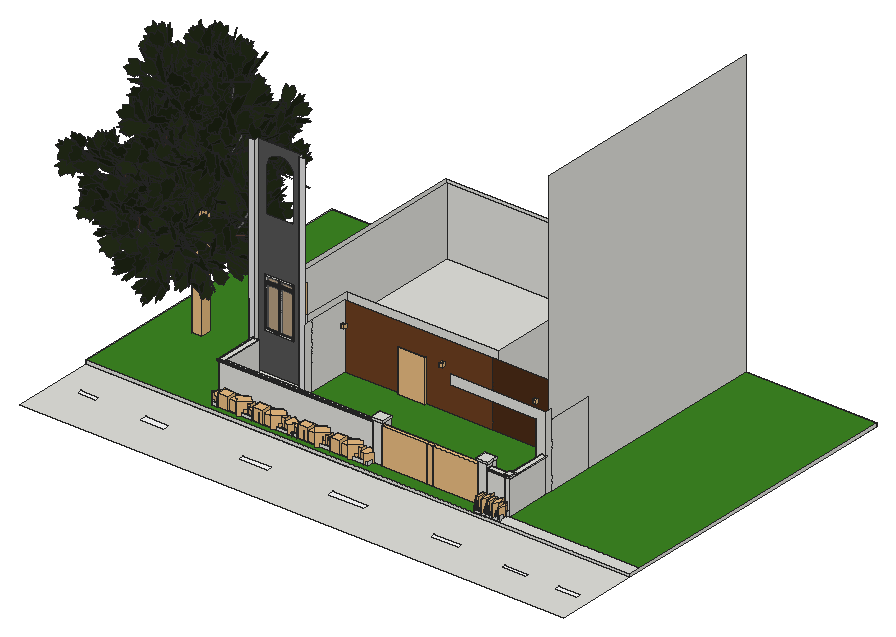
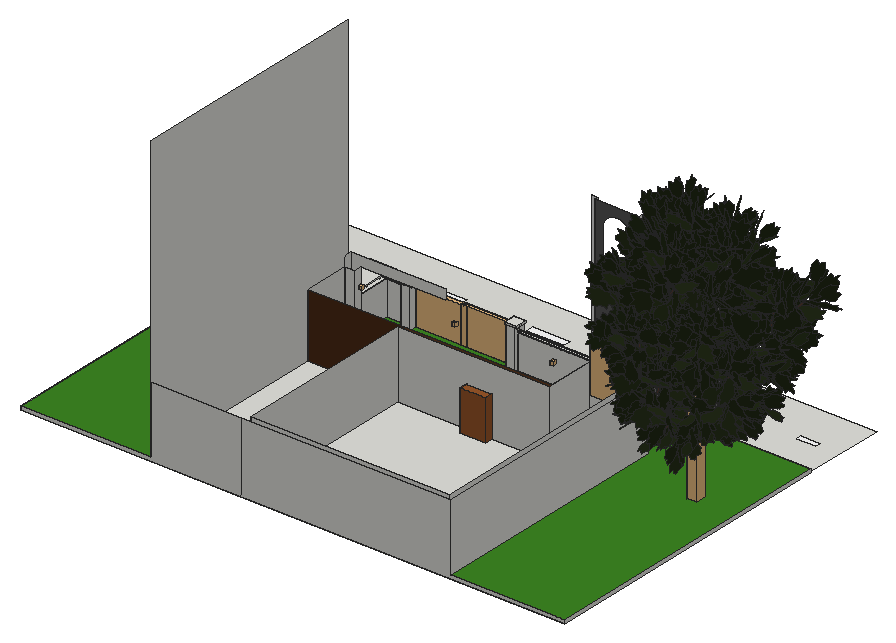
# SketchUp Ruby script. Lengths in inches.
U = 1.inch
M = Sketchup.active_model
def pt(a) = Geom::Point3d.new(a.map { |v| v * U })
def face(e, loops, mat)
  f = e.add_face(loops[0].map { |a| pt(a) })
  loops[1..].each { |l| e.add_face(l.map { |a| pt(a) }).erase! }
  f.material = f.back_material = mat if mat
  f
end
# faces: each face lists its corners as indices into pts; further lists are holes
def faces(e, pts, list, mat = nil) = list.each { |f| face(e, (f[0].is_a?(Array) ? f : [f]).map { |l| l.map { |i| pts[i] } }, mat) }
# xy, xz, yz: faces in a plane at the given z, y or x. An outline is a flat list of corners, or four numbers for a rectangle; further outlines are holes
def ring(l) = l.size == 4 ? [[l[0], l[1]], [l[2], l[1]], [l[2], l[3]], [l[0], l[3]]] : l.each_slice(2).to_a
def flat(e, list, mat, &to3) = list.each { |f| face(e, (f[0].is_a?(Array) ? f : [f]).map { |l| ring(l).map { |u, v| to3.(u, v) } }, mat) }
def xy(e, z, list, mat = nil) = flat(e, list, mat) { |x, y| [x, y, z] }
def xz(e, y, list, mat = nil) = flat(e, list, mat) { |x, z| [x, y, z] }
def yz(e, x, list, mat = nil) = flat(e, list, mat) { |y, z| [x, y, z] }
def lines(e, pts, list) = list.each { |a, b| e.add_line(pt(pts[a]), pt(pts[b])) }
# prism: a flat outline (further loops are holes) pulled along v
def prism(e, loops, v, mat = nil)
  f = face(e, loops, mat); d = Geom::Vector3d.new(v.map { |x| x * U })
  f.pushpull(f.normal.samedirection?(d) ? d.length : -d.length)
end
def box(e, o, s, mat = nil) = prism(e, [[o, [o[0] + s[0], o[1], o[2]], [o[0] + s[0], o[1] + s[1], o[2]], [o[0], o[1] + s[1], o[2]]]], [0, 0, s[2]], mat)
def at(x, y, z, deg = 0) = Geom::Transformation.translation(pt([x, y, z])) * Geom::Transformation.rotation(ORIGIN, Z_AXIS, deg.degrees)
def axes(o, x, y, z) = Geom::Transformation.new([*x, 0, *y, 0, *z, 0, *pt(o).to_a, 1])
def part(name) = M.definitions.add(name)
# library, detail: a bought-in or finely detailed component or shape, given as its bounding box
def library(name, o, s) = part(name).tap { |d| box(d.entities, o, s) }
def detail(e, o, s) = box(e.add_group.entities, o, s)
def put(e, d, t, mat = nil) = e.add_instance(d, t).tap { |i| i.material = mat if mat }
def group(e, t, mat = nil) = e.add_group.tap { |g| g.transformation = t; g.material = mat if mat }.entities
root = M.entities
M.materials.add("Color_2").color = [255, 255, 255]
M.materials.add("Green ash – green texture").color = [33, 41, 22]
M.materials.add("Material__1").color = [95, 70, 46]
M.materials.add("[Color M00]").color = [60, 133, 34]
M.materials.add("[Color M01]").color = [226, 226, 226]
M.materials.add("[Color M06]").color = [86, 86, 86]
M.materials.add("[Color_005]1").color = [114, 114, 114]
M.materials.add("[Color_D09]").color = [86, 59, 49]
M.materials.add("[Translucent Glass Gray]").color = [128, 128, 128]
M.materials["[Translucent Glass Gray]"].alpha = 0.5
M.materials.add("[Wood Cherry Original]").color = [152, 86, 42]
M.materials.add("[Wood Veneer 01]").color = [76, 44, 23]
M.materials.add("[Wood Veneer 01]1").color = [109, 63, 33]
c1 = part("Component\#13")
xz(c1.entities,0,[[2.54,0,9.87,0.64,10.99,2.07,11.4,3.42,15.13,2.28,14.48,4.31,16.14,5.21,16.14,6.08,19.81,7.28,19.6,9.67,17.45,11.49,17.45,12.16,18.82,14.37,17.48,14.37,14.41,13.66,14.41,15.23,12.5625,17.49,9.84,15.21,8.9,13.85,7.74,13.625,7.35,12.68,6.87,13.02,6.35,12.27,5.92,10.47,4.2,7.42,2.84,6.89,0,2.38,0.07,1.59,2.8125,4.94,3.37,3.59,2.54,3.37,2.12,2.22]],"Green ash – green texture")
c2 = part("Component\#14")
xz(c2.entities,0,[[1.1,0,1.61,0,2.73,1.11,4.34,2.72,5.21,6.36,5.85,7.16,6.35,6.9375,6.85,8.05,8.03,8.05,8.625,9.25,10.11,11.7,9.56,13.83,9.56,15.84,7.83,15.84,6.03,14.37,5.31,16.54,4.4375,17.39,1.45,14.31,0,9.15,1.4,5.18,3.01,6.08,1.98,1.39]],"Green ash – green texture")
c3 = part("Component\#16")
put(c3.entities,c1,axes([0,7.77,0],[1,0,0],[0,0.89571,0.44464],[0,-0.44464,0.89571]))
put(c3.entities,c2,axes([2.15,6.37,5.26],[0.57629,-0.80824,0.12095],[0.79263,0.51673,-0.3236],[0.19905,0.28236,0.93843]))
c4 = part("Component\#3")
put(c4.entities,c3,axes([-4.97,-3.22,4.05],[0.69883,-0.69034,0.18725],[0.53248,0.3273,-0.7806],[0.47759,0.64522,0.59632]))
c5 = part("Component\#4")
put(c5.entities,c4,axes([0,5.2,2.2],[1,0,0],[0,0.90259,0.43051],[0,-0.43051,0.90259]))
c6 = part("leaf group 2")
put(c6.entities,c5,axes([-11.99,4.41,-4.35],[2.22014,-0.82385,1.14017],[1.36501,1.77637,-1.37441],[-0.33979,1.75315,1.92841]))
c7 = part("Component\#5")
put(c7.entities,c6,axes([-5.27,11.65,1.68],[-0.48323,0.10636,-0.43072],[-0.11515,-0.64511,-0.03012],[-0.42845,0.05342,0.49388]))
c8 = part("Component\#2")
xz(c8.entities,0,[[0.64,0,0,0.1875,4.21,2.81,8.59,4.11,12.8,4.11,19.57,2.81,12.8,3.73,8.59,3.73,4.21,2.3125]],"[Color_D09]")
c9 = part("Leafy twig")
put(c9.entities,c7,axes([23.53,12.57,24.85],[0.06536,-0.90475,-0.42089],[0.61791,-0.2945,0.72901],[-0.78353,-0.30772,0.53981]))
put(c9.entities,c7,axes([22.7,12.25,24.83],[-0.47146,-0.89493,0.11311],[0.80135,-0.48549,-0.35888],[0.36776,-0.0521,0.90651]))
put(c9.entities,c7,axes([24.25,0.65,20.83],[0.8253,-0.50372,0.24924],[0.23848,0.71461,0.65749],[-0.51157,-0.48438,0.71194]))
put(c9.entities,c7,axes([23.54,-2.45,18.63],[0.04689,-0.92492,0.3511],[0.72122,-0.28285,-0.64421],[0.71641,0.2674,0.65188]))
put(c9.entities,c7,axes([22.39,16.15,27.04],[-0.5311,-0.82173,0.2419],[0.41574,0.01583,0.89559],[-0.77461,0.50499,0.40813]))
put(c9.entities,c8,axes([22.76,-5.09,13.48],[0,1.66539,0.44624],[-1.72414,0,0],[0,-0.44624,1.66539]))
c10 = part("Bare twig")
p = [[0,0,0.13],[0.41,0.77,0],[4.07,2.79,10.125],[3.73,2.15,10.23],[7.66,4.77,23.875],[7.4,4.27,23.96],
  [8.6875,5.26,35.99],[8.5,4.91,36.05],[8.32,4.9375,46.95],[8.21,4.74,46.98]]
faces(c10.entities,p,[[0,1,2,3],[3,2,4,5],[4,6,7,5],[6,8,9,7]],"[Color_005]1")
c11 = part("Leafy twig \#1")
put(c11.entities,c10,axes([3.13,0.17,-0.45],[3.38032,6.88592,0.52481],[-5.85488,3.97559,0.303],[0,-1.35912,3.54524]))
put(c11.entities,c7,axes([0.37,31.375,148.94],[0.47772,0.64064,-1.51139],[2.85768,-0.62659,0.20284],[-0.43926,-3.3797,-0.3241]))
c12 = part("Tree branch")
put(c12.entities,c9,axes([28.11,72.66,46.26],[0.77413,-0.41274,-0.47998],[0.6311,0.56229,0.53435],[0.04934,-0.71657,0.69577]))
put(c12.entities,c9,axes([31.25,3.94,9.17],[0.73236,0.67893,0.05208],[-0.46223,0.55185,-0.69413],[-0.5,0.48428,0.71797]))
put(c12.entities,c9,axes([20.16,84.84,57.95],[0.96628,0.19619,0.16678],[-0.2575,0.73909,0.62245],[-0.00115,-0.6444,0.76469]))
put(c12.entities,c9,axes([30.13,29.18,11.93],[0.86603,0.2796,0.41452],[0,0.82904,-0.55919],[-0.5,0.48428,0.71797]))
put(c12.entities,c9,axes([47.67,28.63,-3.7],[0.1205,-0.71255,0.69119],[0.96646,0.24327,0.08231],[-0.2268,0.65809,0.71797]))
put(c12.entities,c9,axes([48.76,50.64,76.31],[-0.6716,0.46861,-0.57389],[0.01402,0.78248,0.62252],[0.74078,0.41004,-0.53209]))
put(c12.entities,c11,axes([42.34,0,10.34],[0.39368,0,0],[0,0.22544,-0.24092],[0,0.54032,0.50562]))
put(c12.entities,c9,axes([64.51,80.82,101.08],[-0.99604,0.06562,-0.06004],[-0.0106,0.58266,0.81265],[0.08831,0.81006,-0.57966]))
c13 = library("Tree trunk",[-6.35,9.4375,-76.57],[12.56,13.68,315.77])
c14 = part("Tree branch \#2")
put(c14.entities,c9,axes([-3.64,36.17,23.18],[0.95801,0.10249,0.26779],[-0.28581,0.41631,0.86313],[-0.02302,-0.90343,0.42812]))
put(c14.entities,c9,axes([13.16,55.79,39.92],[0.70711,-0.61725,0.34497],[0,0.48786,0.87292],[-0.70711,-0.61725,0.34497]))
put(c14.entities,c11,axes([18.8125,5.17,0.46],[0.25503,0,0],[0,0.20007,-0.0752],[0,0.16866,0.44872]))
put(c14.entities,c9,axes([23.62,-10.17,21.5],[-0.56253,0.81775,0.12181],[0.38738,0.13053,0.91263],[0.73041,0.56057,-0.39021]))
put(c14.entities,c9,axes([45.18,27.18,68.96],[-0.96593,-0.22593,0.12627],[0.12295,0.02876,0.992],[-0.22775,0.97372,0]))
c15 = part("Tree branch \#3")
put(c15.entities,c11,axes([21.47,3.93,0.22],[0.25503,0,0],[0,0.21068,-0.03601],[0,0.08077,0.47252]))
put(c15.entities,c9,axes([-4.05,13.6875,55.34],[0.70711,0.70373,-0.069],[0,0.09758,0.99523],[0.70711,-0.70373,0.069]))
put(c15.entities,c9,axes([6.52,33.54,18.07],[0.92587,-0.37604,0.03687],[0,0.09758,0.99523],[-0.37784,-0.92145,0.09035]))
c16 = part("Tree branch \#1")
put(c16.entities,c9,axes([26.17,74.02,40.56],[0.25882,-0.64004,0.72344],[0,0.74896,0.66262],[-0.96593,-0.1715,0.19384]))
put(c16.entities,c9,axes([6.38,24.03,55.81],[-0.04786,0.8645,-0.50035],[0.15558,0.50126,0.85119],[0.98666,-0.03711,-0.15849]))
put(c16.entities,c11,axes([17.68,0,1.01],[0.32282,0,0],[0,0.21407,-0.16545],[0,0.37107,0.48011]))
put(c16.entities,c9,axes([-9.1875,31.15,28.07],[0.82314,0.37626,-0.42529],[0,0.74896,0.66262],[0.56784,-0.54543,0.61649]))
put(c16.entities,c9,axes([0.54,-12.07,9.94],[0.19622,0.90478,-0.37799],[-0.67396,0.40444,0.61823],[0.71224,0.13344,0.68914]))
put(c16.entities,c9,axes([7.34,9.15,39.57],[0.05153,0.73872,-0.67204],[0.38679,0.60565,0.6954],[0.92072,-0.29578,-0.25452]))
put(c16.entities,c9,axes([36.2,51.23,15.73],[-0.18626,-0.35374,0.91661],[-0.31641,0.90483,0.2849],[-0.93016,-0.23696,-0.28046]))
c17 = part("Tree")
put(c17.entities,c12,axes([-22.29,52.36,216.76],[0.38964,-1.07313,-0.10036],[1.06809,0.37236,0.19631],[-0.13881,-0.14712,1.22884]))
put(c17.entities,c12,axes([59.83,6.78,230.57],[-1.28826,-0.23008,-0.3647],[0.05148,-1.22938,0.51215],[-0.34663,0.55136,1.25774]))
put(c17.entities,c13,axes([-2.16,-18.04,104.22],[1.30157,0,0],[0,1.30157,0],[0,0,1.36111]))
put(c17.entities,c12,axes([-55.8,4.2,115.32],[1.30157,0,0],[0,1.29536,0.19359],[0,-0.26855,1.38538]))
put(c17.entities,c12,axes([5.36,-52.22,156.04],[-0.23532,1.19719,-0.71362],[-1.32974,0,0.39335],[0.40758,0.6912,1.23603]))
put(c17.entities,c14,axes([-20.09,22.57,317.7],[0,-1.33697,0],[1.33697,0,0],[0,0,1.4573]))
put(c17.entities,c12,axes([44.2,-31.84,172.82],[-1.11894,0.85085,0],[-0.85085,-1.11894,0],[0,0,1.53221]))
put(c17.entities,c12,axes([-10.2,63.7,119.93],[0.28716,-1.46366,0],[1.41378,0.27737,0.38604],[-0.41292,-0.08101,1.5704]))
put(c17.entities,c12,axes([-29.03,-40.72,232.79],[0.5211,0.98898,-0.38718],[-1.02974,0.58664,0.11255],[0.35577,0.28216,1.19957]))
put(c17.entities,c12,axes([44.92,21.7,135.38],[-1.05627,-0.44294,0],[0.44294,-1.05627,0],[0,0,1.24847]))
put(c17.entities,c14,axes([-32.94,-0.59,304.82],[1.2814,-0.22825,0],[0.22825,1.2814,0],[0,0,1.41871]))
put(c17.entities,c14,axes([0.6,-31.29,315.98],[0.13082,1.33422,0],[-1.33422,0.13082,0],[0,0,1.46127]))
put(c17.entities,c14,axes([21.3,1.66,315.16],[-1.25722,0.32198,-0.09905],[-0.32539,-1.26867,0.00612],[-0.08719,0.09194,1.40547]))
put(c17.entities,c15,axes([-19,30.84,372.72],[0.65078,-1.12719,0],[1.12719,0.65078,0],[0,0,1.41871]))
put(c17.entities,c15,axes([14.39,-16.125,357],[-0.73695,1.06095,0.15933],[-1.03698,-0.75397,0.2242],[0.29981,0,1.38667]))
put(c17.entities,c16,axes([-5.9,-20.03,270.39],[0,1.47598,0],[-1.4157,0,0.41751],[0.45509,0,1.54311]))
put(c17.entities,c16,axes([-18.4375,22.18,263.88],[0.84243,-1.42226,-0.32685],[1.40385,0.7063,0.64743],[-0.37678,-0.54841,1.68147]))
put(c17.entities,c16,axes([-29.32,4.9,283.41],[1.35363,0,0],[0,1.33841,0.20242],[0,-0.22063,1.45887]))
put(c17.entities,c16,axes([17.31,11.65,257.52],[-1.14969,-0.5642,-0.25322],[0.46017,-1.12719,0.50159],[-0.40066,0.32434,1.3027]))
put(c17.entities,c16,axes([16.3,15.3125,240.45],[-0.98541,-0.85203,0.68095],[1.00747,-1.01506,0.22317],[0.31818,0.5753,1.40228]))
put(c17.entities,c12,axes([-46.75,22.93,206.12],[1.08363,-0.37101,0],[0.37101,1.08363,0],[0,0,1.24847]))
put(c17.entities,c12,axes([41.1,-35.18,99.125],[-1.05556,0.85173,0.25344],[-0.84493,-1.04965,0.12953],[0.39153,-0.09409,1.38106]))
c18 = library("door (1)",[38.93,25.48,0],[40,9.94,82.68])
c19 = part("Untitled (5)")
xy(c19.entities,0,[[[158.81,26.5625,306.06,993.3125],[226.57,518.17,239.57,583.92],[225.28,357.51,237.28,411.51],[222.61,182.28,236.36,226.53],[239.71,931.55,251.46,972.3],[233.64,703.93,242.14,755.18],[240.05,835.03,248.8,880.53],[222.04,66.5,231.29,100.5]]])
xy(c19.entities,0,[[222.04,66.5,231.29,100.5],[222.61,182.28,236.36,226.53],[225.28,357.51,237.28,411.51],[226.57,518.17,239.57,583.92],[233.64,703.93,242.14,755.18],
  [240.05,835.03,248.8,880.53],[239.71,931.55,251.46,972.3]],"Color_2")
c20 = library("Areca palm plant",[0,0,0],[49.1,36.6,54.46])
c21 = library("Group20\#1",[-20.81,-17.08,3.79],[39.86,39.43,37.51])
c22 = library("Group\#74",[-84.69,-90.07,-0.36],[176.51,175.13,171.4])
c23 = library("Group\#130",[-7.34,-1.2,0],[38.67,35.81,49.04])
c24 = library("Group38\#2",[14.01,28.44,-23.43],[18.58,18.32,38.89])
c25 = part("Group\#11")
put(c25.entities,c20,axes([-6.2,56.6,6.08],[0.45017,-0.56191,0],[0.66137,0.52986,0],[0,0,0.72]))
put(c25.entities,c20,axes([-6.2,158.41,6.08],[0.45017,-0.56191,0],[0.66137,0.52986,0],[0,0,0.72]))
put(c25.entities,c21,axes([18.97,181.79,4.77],[0,0.85,0],[-0.85,0,0],[0,0,0.85]))
put(c25.entities,c22,axes([14.93,71.3,6.05],[-0.04961,-0.08593,0],[0.08593,-0.04961,0],[0,0,0.10522]))
put(c25.entities,c22,axes([14.93,91.37,6.05],[-0.04961,-0.08593,0],[0.08593,-0.04961,0],[0,0,0.10522]))
put(c25.entities,c21,axes([18.97,79.98,4.77],[0,0.85,0],[-0.85,0,0],[0,0,0.85]))
put(c25.entities,c23,axes([24.9375,191.72,8],[0,0.79,0],[-0.79,0,0],[0,0,0.79]))
put(c25.entities,c22,axes([17.19,223.04,6.07],[-0.08133,-0.14087,0],[0.14087,-0.08133,0],[0,0,0.1725]))
put(c25.entities,c23,axes([24.9375,89.91,8],[0,0.79,0],[-0.79,0,0],[0,0,0.79]))
put(c25.entities,c22,axes([14.93,44.05,6.05],[-0.04961,-0.08593,0],[0.08593,-0.04961,0],[0,0,0.10522]))
put(c25.entities,c22,axes([14.93,145.87,6.05],[-0.04961,-0.08593,0],[0.08593,-0.04961,0],[0,0,0.10522]))
put(c25.entities,c24,axes([-4.1,100.66,28.17],[0.8848,0,0],[0,0.94674,0],[0,0,0.85826]))
put(c25.entities,c22,axes([14.93,173.12,6.05],[-0.04961,-0.08593,0],[0.08593,-0.04961,0],[0,0,0.10522]))
put(c25.entities,c24,axes([-4.1,-1.15,28.17],[0.8848,0,0],[0,0.94674,0],[0,0,0.85826]))
put(c25.entities,c22,axes([17.19,121.23,6.07],[-0.08133,-0.14087,0],[0.14087,-0.08133,0],[0,0,0.1725]))
put(c25.entities,c22,axes([14.93,193.18,6.05],[-0.04961,-0.08593,0],[0.08593,-0.04961,0],[0,0,0.10522]))
put(c25.entities,c22,axes([17.19,15.79,6.07],[-0.08133,-0.14087,0],[0.14087,-0.08133,0],[0,0,0.1725]))
g1 = group(c25.entities,at(0,0,0))
xy(g1,0,[[0,0,6,234.8],[30,0,36,234.8]])
xy(g1,3,[[6,0,30,234.8]])
xy(g1,7,[[6,5,30,229.8]],"Material__1")
xy(g1,15,[[[0,0,36,234.8],[6,5,30,229.8]]])
xz(g1,0,[[0,0,6,0,6,3,30,3,30,0,36,0,36,15,0,15]])
xz(g1,5,[[6,7,30,15]])
xz(g1,229.8,[[6,7,30,15]])
xz(g1,234.8,[[0,0,0,15,36,15,36,0,30,0,30,3,6,3,6,0]])
yz(g1,0,[[0,0,234.8,15]])
yz(g1,6,[[0,0,234.8,3],[5,7,229.8,15]])
yz(g1,30,[[0,0,234.8,3],[5,7,229.8,15]])
yz(g1,36,[[0,0,234.8,15]])
c26 = library("SLIDING GATE",[0,0,0],[90.55,6.89,64.23])
c27 = library("Curtains",[0,0,0],[121.73,8.19,117.22])
c28 = part("Group\#3")
xy(c28.entities,0,[[0,0,32.48,1.97]])
xy(c28.entities,0.98,[[0.98,0,31.5,0.98],[0.98,0.98,31.5,1.97]])
xy(c28.entities,8.86,[[0.98,0,31.5,0.98],[0.98,0.98,31.5,1.97]])
xy(c28.entities,9.84,[[0,0,32.48,1.97]])
xz(c28.entities,0,[[[0,0,32.48,9.84],[0.98,0.98,31.5,8.86]]])
xz(c28.entities,0.98,[[0.98,0.98,31.5,8.86]],"[Translucent Glass Gray]")
xz(c28.entities,1.97,[[[0,0,32.48,9.84],[0.98,0.98,31.5,8.86]]])
yz(c28.entities,0,[[0,0,1.97,9.84]])
yz(c28.entities,0.98,[[0,0.98,0.98,8.86],[0.98,0.98,1.97,8.86]])
yz(c28.entities,31.5,[[0,0.98,0.98,8.86],[0.98,0.98,1.97,8.86]])
yz(c28.entities,32.48,[[0,0,1.97,9.84]])
c29 = part("Group\#4")
xy(c29.entities,0,[[0,0,32.48,1.97]])
xy(c29.entities,0.98,[[0.98,0,31.5,0.98],[0.98,0.98,31.5,1.97]])
xy(c29.entities,71.85,[[0.98,0,31.5,0.98],[0.98,0.98,31.5,1.97]])
xy(c29.entities,72.83,[[0,0,32.48,1.97]])
xz(c29.entities,0,[[[0,0,32.48,72.83],[0.98,0.98,31.5,71.85]]])
xz(c29.entities,0.98,[[0.98,0.98,31.5,71.85]],"[Translucent Glass Gray]")
xz(c29.entities,1.97,[[[0,0,32.48,72.83],[0.98,0.98,31.5,71.85]]])
yz(c29.entities,0,[[0,0,1.97,72.83]])
yz(c29.entities,0.98,[[0,0.98,0.98,71.85],[0.98,0.98,1.97,71.85]])
yz(c29.entities,31.5,[[0,0.98,0.98,71.85],[0.98,0.98,1.97,71.85]])
yz(c29.entities,32.48,[[0,0,1.97,72.83]])
c30 = part("FIXED+GLASS+WINDOW+WITH+TRANSOM")
g2 = group(c30.entities,at(0,0,0))
xy(g2,0,[[0,0,70.86,3.9375]])
xy(g2,1.97,[[1.97,0,34.45,0.98],[36.42,0,68.9,3.9375],[1.97,2.95,34.45,3.9375]])
xy(g2,86.61,[[1.97,0,34.45,3.9375],[34.45,0,36.42,3.9375],[36.42,0,68.9,3.9375]])
xy(g2,88.58,[[0,0,70.86,3.9375]])
xz(g2,0,[[[0,0,70.86,88.58],[1.97,1.97,34.45,86.61],[36.42,1.97,68.9,86.61]]])
xz(g2,3.9375,[[[0,0,70.86,88.58],[1.97,1.97,34.45,86.61],[36.42,1.97,68.9,86.61]]])
yz(g2,0,[[0,0,3.9375,88.58]])
yz(g2,1.97,[[0,1.97,3.9375,74.8],[0,76.77,3.9375,86.61]])
yz(g2,34.45,[[0,1.97,3.9375,86.61]])
yz(g2,36.42,[[0,1.97,3.9375,86.61]])
yz(g2,68.9,[[0,1.97,3.9375,86.61]])
yz(g2,70.86,[[0,0,3.9375,88.58]])
g3 = group(g2,at(1.97,0,74.8))
box(g3,[0,0,0],[66.93,3.9375,1.97])
put(g2,c28,at(1.97,0.98,76.77))
put(g2,c28,at(36.42,0.98,76.77))
put(g2,c29,at(1.97,0.98,1.97))
put(g2,c29,at(36.42,0.98,1.97))
c31 = library("SPOT",[0,0,1.68],[5.4375,5.4375,6.28])
xy(root,0,[[88.81,147.25,664.24,694.43],[664.24,147.25,1057.24,694.43]])
xy(root,6,[[784.82,147.25,817.96,170.11],[817.96,147.25,1057.24,168.49],[817.96,168.49,817.96,170.11,784.82,170.11,784.82,179.52,818.2,179.52,818.2,249.36,825.43,249.36,825.43,168.49],[581.36,170.11,598.29,188.93],[768.57,170.11,784.82,188.93],
  [299.79,178.93,299.79,256.61,308.67,256.61,308.67,183.93,581.36,183.93,581.36,178.93],[301.28,272.46,383.72,272.46,383.72,358.66,488.02,358.66,488.02,372.15,532.64,372.15,532.64,358.66,655.02,358.66,655.02,685.21,301.28,685.21],[488.02,358.66,532.64,372.15]])
xy(root,6,[[88.81,147.25,784.82,147.25,784.82,170.11,768.57,170.11,768.57,188.93,784.82,188.93,784.82,179.52,818.2,179.52,818.2,249.36,808.1,249.36,808.1,263.24,825.43,263.24,825.43,345.71,532.64,345.71,532.64,358.66,488.02,358.66,488.02,345.71,390.34,345.71,390.34,256.61,308.67,256.61,308.67,183.93,581.36,183.93,581.36,188.93,598.29,188.93,598.29,170.11,581.36,170.11,581.36,178.93,299.79,178.93,299.79,256.61,292.06,256.61,292.06,694.43,88.81,694.43],[825.43,168.49,1057.24,694.43]],"[Color M00]")
xy(root,15.375,[[302.78,256.61,380.53,263.24]])
xy(root,66,[[784.82,168.36,784.82,170.11,817.96,170.11,817.96,168.49,825.43,168.49,825.43,168.36],[825.43,168.36,827.18,170.11],[817.96,168.49,825.43,170.11],[784.82,170.11,784.82,179.52,818.2,179.52,818.2,249.36,825.43,249.36,825.43,170.11],[825.43,170.11,827.18,249.36],
  [298.04,177.18,299.79,178.93],[299.79,177.18,581.36,178.93],[298.04,178.93,299.79,256.61],[299.79,178.93,299.79,256.61,308.67,256.61,308.67,183.93,581.36,183.93,581.36,178.93]])
xy(root,67.75,[[784.82,168.36,817.26,170.11],[784.82,170.11,817.26,179.52],[298.04,177.18,299.79,178.93],[299.79,177.18,581.36,178.93],[298.04,178.93,299.79,256.61],
  [299.79,178.93,581.36,178.93,581.36,183.93,308.67,183.93,308.67,256.61,299.79,256.61],[818.2,179.52,825.43,249.36],[825.43,179.52,827.18,249.36]])
xy(root,69.9375,[[816.32,167.49,817.26,179.52],[817.26,167.49,827.18,168.36],[817.26,168.36,827.18,179.52]])
xy(root,71.0625,[[816.32,167.49,827.18,179.52]])
xy(root,75.375,[[579.04,167.8,600.61,170.11],[766.26,167.8,787.14,170.11],[579.04,170.11,581.36,178.93],[581.36,170.11,598.29,188.93],[598.29,170.11,600.61,188.93],
  [766.26,170.11,768.57,188.93],[768.57,170.11,784.82,188.93],[784.82,170.11,787.14,179.52],[579.04,178.93,581.36,183.93],[784.82,179.52,787.14,188.93],
  [579.04,183.93,581.36,188.93]])
xy(root,78.2,[[488.02,345.71,532.64,372.15]],"[Wood Cherry Original]")
xy(root,79.0625,[[579.04,167.8,600.61,188.93],[766.26,167.8,787.14,188.93]])
xy(root,81.74,[[314.4,263.24,366.4,272.46]])
xz(root,147.25,[[88.81,0,1057.24,6]])
xz(root,167.49,[[816.32,69.9375,827.18,71.0625]])
xz(root,167.8,[[579.04,75.375,600.61,79.0625],[766.26,75.375,787.14,79.0625]])
xz(root,168.36,[[784.82,66,827.18,66,827.18,69.9375,817.26,69.9375,817.26,67.75,784.82,67.75]])
xz(root,168.49,[[817.96,6,825.43,66]])
xz(root,170.11,[[581.36,6,598.29,75.375],[768.57,6,784.82,75.375],[784.82,6,817.96,66]])
xz(root,177.18,[[298.04,66,299.79,67.75],[299.79,66,581.36,67.75]])
xz(root,178.93,[[299.79,6,581.36,66],[298.04,66,299.79,67.75],[299.79,66,581.36,67.75]])
xz(root,179.52,[[784.82,6,818.2,66],[784.82,66,818.2,67.75],[817.26,67.75,825.43,69.9375],[825.43,67.75,827.18,69.9375],[816.32,69.9375,825.43,71.0625],
  [825.43,69.9375,827.18,71.0625]])
xz(root,183.93,[[308.67,6,581.36,66],[308.67,66,581.36,67.75]])
xz(root,188.93,[[581.36,6,598.29,75.375],[768.57,6,784.82,75.375],[579.04,75.375,600.61,79.0625],[766.26,75.375,787.14,79.0625]])
xz(root,249.36,[[808.1,6,818.2,6,818.2,67.75,825.43,67.75,825.43,138,657.09,138,657.09,120.375,808.1,120.375],[818.2,6,825.43,66],[818.2,66,825.43,67.75],[825.43,66,827.18,67.75]])
xz(root,256.61,[[299.79,6,308.67,6,308.67,15.375,302.78,15.375,302.78,66,299.79,66],[302.78,15.375,308.67,66],[298.04,66,299.79,67.75],[299.79,66,302.78,67.75],[302.78,66,308.67,67.75]])
xz(root,256.61,[[292.06,6,299.79,6,299.79,66,298.04,66,298.04,67.75,302.78,67.75,302.78,384,292.06,384],[308.67,6,390.34,6,390.34,384,380.53,384,380.53,15.375,308.67,15.375]],"[Color M01]")
xz(root,263.24,[[808.1,6,825.43,120.375]])
xz(root,263.24,[[[302.78,15.375,380.53,384],[316.75,267.28,316.75,343.59,317.6,350,320.07,355.97,324,361.09,329.125,365.03,335.1,367.5,341.5,368.34,347.91,367.5,353.875,365.03,359,361.09,362.9375,355.97,365.41,350,366.25,343.59,366.25,267.28],[314.4,81.74,366.4,171.49]]],"[Color M06]")
xz(root,272.46,[[301.28,6,301.28,126,314.4,126,314.4,81.74,366.4,81.74,366.4,126,383.72,126,383.72,6]])
xz(root,345.71,[[655.02,6,825.43,120.375]],"[Wood Veneer 01]")
xz(root,345.71,[[390.34,6,488.02,6,488.02,78.2,532.64,78.2,532.64,6,655.02,6,655.02,120.375,390.34,120.375]],"[Wood Veneer 01]1")
xz(root,358.66,[[383.72,6,655.02,126]])
xz(root,372.15,[[488.02,6,532.64,78.2]],"[Wood Cherry Original]")
xz(root,685.21,[[301.28,6,655.02,126]])
xz(root,694.43,[[88.81,0,88.81,6,292.06,6,292.06,126,664.24,126,664.24,0],[664.24,0,664.24,126,825.43,126,825.43,6,1057.24,6,1057.24,0]])
yz(root,88.81,[[147.25,0,694.43,6]])
yz(root,292.06,[[256.61,6,694.43,126]])
yz(root,298.04,[[177.18,66,178.93,67.75],[178.93,66,256.61,67.75]])
yz(root,299.79,[[178.93,6,256.61,66],[177.18,66,178.93,67.75],[178.93,66,256.61,67.75]])
yz(root,301.28,[[272.46,6,685.21,126]])
yz(root,302.78,[[256.61,15.375,263.24,384]])
yz(root,308.67,[[183.93,6,256.61,66],[183.93,66,256.61,67.75]])
yz(root,314.4,[[263.24,81.74,272.46,171.49]])
yz(root,366.4,[[263.24,81.74,272.46,171.49]])
yz(root,380.53,[[256.61,15.375,263.24,384]])
yz(root,383.72,[[272.46,6,358.66,126]])
yz(root,390.34,[[256.61,6,272.46,120.375],[272.46,6,345.71,120.375]])
yz(root,488.02,[[345.71,6,372.15,78.2]],"[Wood Cherry Original]")
yz(root,532.64,[[345.71,6,372.15,78.2]],"[Wood Cherry Original]")
yz(root,579.04,[[167.8,75.375,178.93,79.0625],[178.93,75.375,183.93,79.0625],[183.93,75.375,188.93,79.0625]])
yz(root,581.36,[[170.11,6,170.11,75.375,178.93,75.375,178.93,67.75,177.18,67.75,177.18,66,178.93,66,178.93,6],[178.93,6,183.93,66],[183.93,6,188.93,75.375],[177.18,66,178.93,67.75],[178.93,66,183.93,67.75],
  [178.93,67.75,183.93,75.375]])
yz(root,598.29,[[170.11,6,188.93,75.375]])
yz(root,600.61,[[167.8,75.375,188.93,79.0625]])
yz(root,655.02,[[358.66,6,685.21,126]])
yz(root,766.26,[[167.8,75.375,188.93,79.0625]])
yz(root,768.57,[[170.11,6,188.93,75.375]])
yz(root,784.82,[[170.11,6,179.52,66],[179.52,6,188.93,75.375],[168.36,66,170.11,67.75],[170.11,66,179.52,67.75],[170.11,67.75,179.52,75.375]])
yz(root,787.14,[[167.8,75.375,179.52,79.0625],[179.52,75.375,188.93,79.0625]])
yz(root,808.1,[[249.36,6,263.24,120.375]])
yz(root,816.32,[[167.49,69.9375,179.52,71.0625]])
yz(root,817.26,[[168.36,67.75,179.52,69.9375]])
yz(root,817.96,[[168.49,6,170.11,66]])
yz(root,818.2,[[179.52,6,249.36,66],[179.52,66,249.36,67.75]])
yz(root,825.43,[[168.49,6,249.36,66],[249.36,6,263.24,138],[345.71,6,694.43,6,694.43,510,256.61,510,256.61,138,263.24,138,263.24,120.375,345.71,120.375],[263.24,6,345.71,120.375]])
yz(root,827.18,[[168.36,66,249.36,66,249.36,67.75,179.52,67.75,179.52,69.9375,168.36,69.9375],[167.49,69.9375,179.52,71.0625]])
yz(root,1057.24,[[147.25,0,694.43,6]])
p = [[825.43,170.11,66],[825.43,170.11,67.75]]
lines(root,p,[[0,1]])
put(root,c17,at(165.7,306.86,-20.03))
put(root,c18,axes([440.17,317.49,-2.45],[1.2,0,0],[0,1,0],[0,0,1]))
put(root,c19,at(63.93,306.06,0,-90))
put(root,c25,axes([447.36,158.41,2.45],[0,0.57,0],[-0.60903,0,0],[0,0,0.57]))
put(root,c25,axes([581.36,158.41,2.45],[0,0.57,0],[-0.57,0,0],[0,0,0.57]))
put(root,c26,at(598.29,169.13,6))
put(root,c26,at(677.8,169.07,6))
put(root,c25,axes([824.66,147.25,7.12],[0,0.57,0],[-0.1907,0,0],[0,0,0.57]))
put(root,c27,axes([290.16,270.24,79.58],[0.71882,0,0],[0,1,0],[0,0,0.79]))
put(root,c30,axes([314.4,263.24,81.74],[0.7338,0,0],[0,1,0],[0,0,1.01318]))
put(root,c31,at(429.89,288.3,113.14))
put(root,c31,at(604.95,288.3,113.14))
put(root,c31,at(771.08,288.3,113.14))
